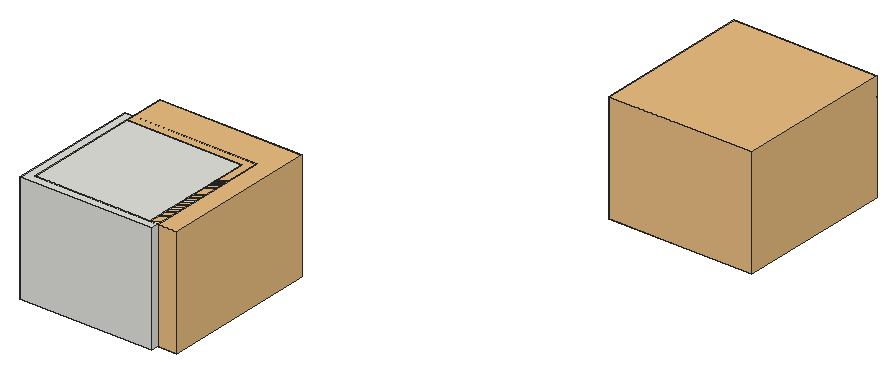
# SketchUp Ruby script. Lengths in inches.
U = 1.inch
M = Sketchup.active_model
def pt(a) = Geom::Point3d.new(a.map { |v| v * U })
def face(e, loops, mat)
  f = e.add_face(loops[0].map { |a| pt(a) })
  loops[1..].each { |l| e.add_face(l.map { |a| pt(a) }).erase! }
  f.material = f.back_material = mat if mat
  f
end
# faces: each face lists its corners as indices into pts; further lists are holes
def faces(e, pts, list, mat = nil) = list.each { |f| face(e, (f[0].is_a?(Array) ? f : [f]).map { |l| l.map { |i| pts[i] } }, mat) }
# xy, xz, yz: faces in a plane at the given z, y or x. An outline is a flat list of corners, or four numbers for a rectangle; further outlines are holes
def ring(l) = l.size == 4 ? [[l[0], l[1]], [l[2], l[1]], [l[2], l[3]], [l[0], l[3]]] : l.each_slice(2).to_a
def flat(e, list, mat, &to3) = list.each { |f| face(e, (f[0].is_a?(Array) ? f : [f]).map { |l| ring(l).map { |u, v| to3.(u, v) } }, mat) }
def xy(e, z, list, mat = nil) = flat(e, list, mat) { |x, y| [x, y, z] }
def xz(e, y, list, mat = nil) = flat(e, list, mat) { |x, z| [x, y, z] }
def yz(e, x, list, mat = nil) = flat(e, list, mat) { |y, z| [x, y, z] }
def lines(e, pts, list) = list.each { |a, b| e.add_line(pt(pts[a]), pt(pts[b])) }
# prism: a flat outline (further loops are holes) pulled along v
def prism(e, loops, v, mat = nil)
  f = face(e, loops, mat); d = Geom::Vector3d.new(v.map { |x| x * U })
  f.pushpull(f.normal.samedirection?(d) ? d.length : -d.length)
end
def box(e, o, s, mat = nil) = prism(e, [[o, [o[0] + s[0], o[1], o[2]], [o[0] + s[0], o[1] + s[1], o[2]], [o[0], o[1] + s[1], o[2]]]], [0, 0, s[2]], mat)
def at(x, y, z, deg = 0) = Geom::Transformation.translation(pt([x, y, z])) * Geom::Transformation.rotation(ORIGIN, Z_AXIS, deg.degrees)
def axes(o, x, y, z) = Geom::Transformation.new([*x, 0, *y, 0, *z, 0, *pt(o).to_a, 1])
def part(name) = M.definitions.add(name)
# library, detail: a bought-in or finely detailed component or shape, given as its bounding box
def library(name, o, s) = part(name).tap { |d| box(d.entities, o, s) }
def detail(e, o, s) = box(e.add_group.entities, o, s)
def put(e, d, t, mat = nil) = e.add_instance(d, t).tap { |i| i.material = mat if mat }
def group(e, t, mat = nil) = e.add_group.tap { |g| g.transformation = t; g.material = mat if mat }.entities
root = M.entities
M.materials.add("Marc_Hair").color = [255, 253, 195]
c1 = library("Glass+Door",[0,0,0],[72,5.22,111.09])
c2 = library("RIDEAUX \#16",[0,0,0],[103.86,7.74,93.57])
c3 = library("Furnished bedroom",[0,0,0],[156.18,171.36,120])
c4 = library("Avation+Styled+Ceiling+Fan_JSB",[-19.77,-29.63,-13.8125],[51.59,58.16,13.8125])
xy(root,0,[[0,0,0,24,9,24,9,9,135,9,135,135,9,135,9,120,0,120,0,144,144,144,144,0]])
xy(root,102,[[0,24,9,120]])
xy(root,120,[[[0,0,144,144],[9,9,135,135]]])
xz(root,0,[[0,0,144,120]])
xz(root,9,[[9,0,135,120]])
xz(root,24,[[0,0,9,102]])
xz(root,120,[[0,0,9,102]])
xz(root,144,[[0,0,144,120]])
yz(root,0,[[0,0,0,120,144,120,144,0,120,0,120,102,24,102,24,0]])
yz(root,144,[[0,0,144,120]])
put(root,c1,axes([-4.41,24,0],[0,1.33741,0],[0.92235,0,0],[0,0,0.92235]))
put(root,c2,axes([21.38,10.63,0],[0,1.18235,0],[-1.18235,0,0],[0,0,1.18235]))
put(root,c3,at(9,9,0))
put(root,c3,at(306.4,425.39,0))
g1 = group(root,at(9,9,120))
xy(g1,-14,[[[0,0,126,126],[24,24,102,102]]])
xy(g1,-12,[[[0,0,126,126],[23.9,23.9,102.1,102]],[23.9,23.9,102,24],[102,23.9,102.1,102],[23.9,24,24,102]])
xy(g1,-10,[[23.9,23.9,102.1,102]])
xy(g1,0,[[0,0,126,126]])
xz(g1,0,[[0,-14,126,-12],[0,-12,126,0]])
xz(g1,23.9,[[23.9,-12,102.1,-10]],"Marc_Hair")
xz(g1,24,[[24,-14,102,-12]])
xz(g1,102,[[24,-14,102,-12]])
xz(g1,102,[[23.9,-12,102.1,-10]],"Marc_Hair")
xz(g1,126,[[0,-14,126,-12],[0,-12,126,0]])
yz(g1,0,[[0,-14,126,-12],[0,-12,126,0]])
yz(g1,23.9,[[23.9,-12,102,-10]],"Marc_Hair")
yz(g1,24,[[24,-14,102,-12]])
yz(g1,102,[[24,-14,102,-12]])
yz(g1,102.1,[[23.9,-12,102,-10]],"Marc_Hair")
yz(g1,126,[[0,-14,126,-12],[0,-12,126,0]])
put(g1,c4,at(58.17,68.65,-10))
g2 = group(g1,at(109.12,60.16,-14),"Marc_Hair")
prism(g2,[[[10.15,8.16,-0.2],[9.28,9.28,-0.2],[8.16,10.15,-0.2],[6.84,10.69,-0.2],[5.4375,10.875,-0.2],[4.03,10.69,-0.2],[2.72,10.15,-0.2],[1.59,9.28,-0.2],[0.73,8.16,-0.2],[0.19,6.84,-0.2],[0,5.4375,-0.2],[0.19,4.03,-0.2],[0.73,2.72,-0.2],[1.59,1.59,-0.2],[2.72,0.73,-0.2],[4.03,0.19,-0.2],[5.4375,0,-0.2],[6.84,0.19,-0.2],[8.16,0.73,-0.2],[9.28,1.59,-0.2],[10.15,2.72,-0.2],[10.69,4.03,-0.2],[10.875,5.4375,-0.2],[10.69,6.84,-0.2]]],[0,0,0.2])
xy(g2,-0.2,[[-96,0,-94.59,0.19,-93.28,0.73,-92.16,1.59,-91.29,2.72,-90.75,4.03,-90.5625,5.4375,-90.75,6.84,-91.29,8.16,-92.16,9.28,-93.28,10.15,-94.59,10.69,-96,10.875,-97.41,10.69,-98.72,10.15,-99.84,9.28,-100.71,8.16,-101.25,6.84,-101.4375,5.4375,-101.25,4.03,-100.71,2.72,-99.84,1.59,-98.72,0.73,-97.41,0.19]])
xy(g2,0,[[-48.66,-51.9375,-47.26,-51.75,-45.94,-51.21,-44.82,-50.35,-43.95,-49.22,-43.41,-47.91,-43.23,-46.5,-43.41,-45.09,-43.95,-43.78,-44.82,-42.66,-45.94,-41.79,-47.26,-41.25,-48.66,-41.0625,-50.07,-41.25,-51.38,-41.79,-52.51,-42.66,-53.37,-43.78,-53.91,-45.09,-54.1,-46.5,-53.91,-47.91,-53.37,-49.22,-52.51,-50.35,-51.38,-51.21,-50.07,-51.75],[-48.66,46.75,-47.26,46.93,-45.94,47.48,-44.82,48.34,-43.95,49.47,-43.41,50.78,-43.23,52.1875,-43.41,53.59,-43.95,54.9,-44.82,56.03,-45.94,56.9,-47.26,57.4375,-48.66,57.625,-50.07,57.4375,-51.38,56.9,-52.51,56.03,-53.37,54.9,-53.91,53.59,-54.1,52.1875,-53.91,50.78,-53.37,49.47,-52.51,48.34,-51.38,47.48,-50.07,46.93]])
p = [[-97.41,0.19,0],[-96,0,0],[-96,0,-0.2],[-97.41,0.19,-0.2],[-94.59,0.19,0],[-94.59,0.19,-0.2],
  [-98.72,0.73,0],[-98.72,0.73,-0.2],[-93.28,0.73,0],[-93.28,0.73,-0.2],[-99.84,1.59,0],[-99.84,1.59,-0.2],
  [-92.16,1.59,0],[-92.16,1.59,-0.2],[-100.71,2.72,0],[-100.71,2.72,-0.2],[-91.29,2.72,0],[-91.29,2.72,-0.2],
  [-101.25,4.03,0],[-101.25,4.03,-0.2],[-90.75,4.03,0],[-90.75,4.03,-0.2],[-101.4375,5.4375,0],[-101.4375,5.4375,-0.2],
  [-90.5625,5.4375,0],[-90.5625,5.4375,-0.2],[-101.25,6.84,0],[-101.25,6.84,-0.2],[-90.75,6.84,0],[-90.75,6.84,-0.2],
  [-100.71,8.16,0],[-100.71,8.16,-0.2],[-91.29,8.16,0],[-91.29,8.16,-0.2],[-99.84,9.28,0],[-99.84,9.28,-0.2],
  [-92.16,9.28,0],[-92.16,9.28,-0.2],[-98.72,10.15,0],[-98.72,10.15,-0.2],[-93.28,10.15,0],[-93.28,10.15,-0.2],
  [-97.41,10.69,0],[-97.41,10.69,-0.2],[-94.59,10.69,0],[-94.59,10.69,-0.2],[-96,10.875,0],[-96,10.875,-0.2],
  [-50.07,-51.75,0.2],[-48.66,-51.9375,0.2],[-48.66,-51.9375,0],[-50.07,-51.75,0],[-47.26,-51.75,0.2],[-47.26,-51.75,0],
  [-51.38,-51.21,0.2],[-51.38,-51.21,0],[-45.94,-51.21,0.2],[-45.94,-51.21,0],[-52.51,-50.35,0.2],[-52.51,-50.35,0],
  [-44.82,-50.35,0.2],[-44.82,-50.35,0],[-53.37,-49.22,0.2],[-53.37,-49.22,0],[-43.95,-49.22,0.2],[-43.95,-49.22,0],
  [-53.91,-47.91,0.2],[-53.91,-47.91,0],[-43.41,-47.91,0.2],[-43.41,-47.91,0],[-54.1,-46.5,0.2],[-54.1,-46.5,0],
  [-43.23,-46.5,0.2],[-43.23,-46.5,0],[-53.91,-45.09,0.2],[-53.91,-45.09,0],[-43.41,-45.09,0.2],[-43.41,-45.09,0],
  [-53.37,-43.78,0.2],[-53.37,-43.78,0],[-43.95,-43.78,0.2],[-43.95,-43.78,0],[-52.51,-42.66,0.2],[-52.51,-42.66,0],
  [-44.82,-42.66,0.2],[-44.82,-42.66,0],[-51.38,-41.79,0.2],[-51.38,-41.79,0],[-45.94,-41.79,0.2],[-45.94,-41.79,0],
  [-50.07,-41.25,0.2],[-50.07,-41.25,0],[-47.26,-41.25,0.2],[-47.26,-41.25,0],[-48.66,-41.0625,0.2],[-48.66,-41.0625,0],
  [-50.07,46.93,0.2],[-48.66,46.75,0.2],[-48.66,46.75,0],[-50.07,46.93,0],[-47.26,46.93,0.2],[-47.26,46.93,0],
  [-51.38,47.48,0.2],[-51.38,47.48,0],[-45.94,47.48,0.2],[-45.94,47.48,0],[-52.51,48.34,0.2],[-52.51,48.34,0],
  [-44.82,48.34,0.2],[-44.82,48.34,0],[-53.37,49.47,0.2],[-53.37,49.47,0],[-43.95,49.47,0.2],[-43.95,49.47,0],
  [-53.91,50.78,0.2],[-53.91,50.78,0],[-43.41,50.78,0.2],[-43.41,50.78,0],[-54.1,52.1875,0.2],[-54.1,52.1875,0],
  [-43.23,52.1875,0.2],[-43.23,52.1875,0],[-53.91,53.59,0.2],[-53.91,53.59,0],[-43.41,53.59,0.2],[-43.41,53.59,0],
  [-53.37,54.9,0.2],[-53.37,54.9,0],[-43.95,54.9,0.2],[-43.95,54.9,0],[-52.51,56.03,0.2],[-52.51,56.03,0],
  [-44.82,56.03,0.2],[-44.82,56.03,0],[-51.38,56.9,0.2],[-51.38,56.9,0],[-45.94,56.9,0.2],[-45.94,56.9,0],
  [-50.07,57.4375,0.2],[-50.07,57.4375,0],[-47.26,57.4375,0.2],[-47.26,57.4375,0],[-48.66,57.625,0.2],[-48.66,57.625,0]]
faces(g2,p,[[0,1,2,3],[1,4,5,2],[6,0,3,7],[4,8,9,5],[10,6,7,11],[8,12,13,9],[14,10,11,15],[12,16,17,13],
  [18,14,15,19],[16,20,21,17],[22,18,19,23],[20,24,25,21],[26,22,23,27],[24,28,29,25],[30,26,27,31],[28,32,33,29],
  [34,30,31,35],[32,36,37,33],[38,34,35,39],[36,40,41,37],[42,38,39,43],[40,44,45,41],[46,42,43,47],[44,46,47,45],
  [48,49,50,51],[49,52,53,50],[54,48,51,55],[52,56,57,53],[58,54,55,59],[56,60,61,57],[62,58,59,63],[60,64,65,61],
  [66,62,63,67],[64,68,69,65],[70,66,67,71],[68,72,73,69],[74,70,71,75],[72,76,77,73],[78,74,75,79],[76,80,81,77],
  [82,78,79,83],[80,84,85,81],[86,82,83,87],[84,88,89,85],[90,86,87,91],[88,92,93,89],[94,90,91,95],[92,94,95,93],
  [96,97,98,99],[97,100,101,98],[102,96,99,103],[100,104,105,101],[106,102,103,107],[104,108,109,105],[110,106,107,111],[108,112,113,109],
  [114,110,111,115],[112,116,117,113],[118,114,115,119],[116,120,121,117],[122,118,119,123],[120,124,125,121],[126,122,123,127],[124,128,129,125],
  [130,126,127,131],[128,132,133,129],[134,130,131,135],[132,136,137,133],[138,134,135,139],[136,140,141,137],[142,138,139,143],[140,142,143,141]])
